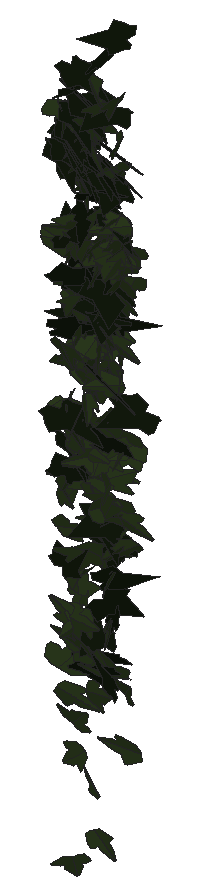
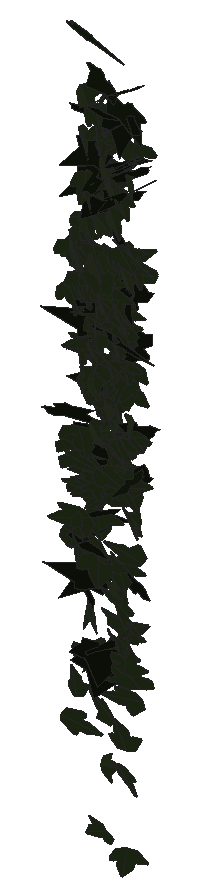
# SketchUp Ruby script. Lengths in millimetres.
U = 1.mm
M = Sketchup.active_model
def pt(a) = Geom::Point3d.new(a.map { |v| v * U })
def face(e, loops, mat)
  f = e.add_face(loops[0].map { |a| pt(a) })
  loops[1..].each { |l| e.add_face(l.map { |a| pt(a) }).erase! }
  f.material = f.back_material = mat if mat
  f
end
# faces: each face lists its corners as indices into pts; further lists are holes
def faces(e, pts, list, mat = nil) = list.each { |f| face(e, (f[0].is_a?(Array) ? f : [f]).map { |l| l.map { |i| pts[i] } }, mat) }
# xy, xz, yz: faces in a plane at the given z, y or x. An outline is a flat list of corners, or four numbers for a rectangle; further outlines are holes
def ring(l) = l.size == 4 ? [[l[0], l[1]], [l[2], l[1]], [l[2], l[3]], [l[0], l[3]]] : l.each_slice(2).to_a
def flat(e, list, mat, &to3) = list.each { |f| face(e, (f[0].is_a?(Array) ? f : [f]).map { |l| ring(l).map { |u, v| to3.(u, v) } }, mat) }
def xy(e, z, list, mat = nil) = flat(e, list, mat) { |x, y| [x, y, z] }
def xz(e, y, list, mat = nil) = flat(e, list, mat) { |x, z| [x, y, z] }
def yz(e, x, list, mat = nil) = flat(e, list, mat) { |y, z| [x, y, z] }
def lines(e, pts, list) = list.each { |a, b| e.add_line(pt(pts[a]), pt(pts[b])) }
# prism: a flat outline (further loops are holes) pulled along v
def prism(e, loops, v, mat = nil)
  f = face(e, loops, mat); d = Geom::Vector3d.new(v.map { |x| x * U })
  f.pushpull(f.normal.samedirection?(d) ? d.length : -d.length)
end
def box(e, o, s, mat = nil) = prism(e, [[o, [o[0] + s[0], o[1], o[2]], [o[0] + s[0], o[1] + s[1], o[2]], [o[0], o[1] + s[1], o[2]]]], [0, 0, s[2]], mat)
def at(x, y, z, deg = 0) = Geom::Transformation.translation(pt([x, y, z])) * Geom::Transformation.rotation(ORIGIN, Z_AXIS, deg.degrees)
def axes(o, x, y, z) = Geom::Transformation.new([*x, 0, *y, 0, *z, 0, *pt(o).to_a, 1])
def part(name) = M.definitions.add(name)
# library, detail: a bought-in or finely detailed component or shape, given as its bounding box
def library(name, o, s) = part(name).tap { |d| box(d.entities, o, s) }
def detail(e, o, s) = box(e.add_group.entities, o, s)
def put(e, d, t, mat = nil) = e.add_instance(d, t).tap { |i| i.material = mat if mat }
def group(e, t, mat = nil) = e.add_group.tap { |g| g.transformation = t; g.material = mat if mat }.entities
root = M.entities
M.materials.add("efeu1").color = [18, 25, 13]
M.materials.add("efeu2").color = [43, 57, 29]
c1 = part("ivyleaf_10")
p = [[0,12.8,-0.8],[-1.5,51.3,-10.9],[-4.9,51,-11.6],[-13.6,26.5,-7.3],[-13.2,15.9,-4.6],[-21.1,19.3,-7.2],
  [-29.5,16.3,-8.3],[-29.2,8.3,-6.2],[-19.7,-9.8,0.5],[-7.6,-13,4],[1,-12.2,5.8],[-0.4,51.1,-11.1],
  [-1.5,51.1,-10.9],[1,-12.4,5.9],[16.9,-12.4,3.5],[35.1,9.1,-5.1],[35,12.9,-6.1],[20.5,16.4,-4.9],
  [15.8,15,-3.8],[15.3,27.6,-7.1],[12.8,31.3,-7.8]]
faces(c1.entities,p,[[0,1,2,3,4,5,6,7,8,9,10],[11,12,0,13,14,15,16,17,18,19,20]],"efeu2")
c2 = part("ivyleaf_9")
p = [[39.1,54.8,31.7],[34.5,51.8,30.2],[-5.3,25.2,17.3],[-17.9,28.3,20.9],[-21.6,21.7,17],[-20.2,4.3,5.3],
  [-22.9,-0.3,2.5],[-17.1,-4,-0.6],[-2,-2.1,-1.2],[-0.7,-15.4,-10.1],[16.6,-22.3,-16.7],[21.1,-15.1,-12.5],
  [32.7,-10.7,-11],[46.1,-1.8,-6.6],[30.8,11.2,3.8]]
faces(c2.entities,p,[[0,1,2,3,4,5,6,7,8,9,10,11,12,13,14]],"efeu1")
put(root,c1,axes([1785.9,1014.5,372.7],[-1.32384,0.17322,0.04012],[0.07345,-0.01106,0.71683],[0.33033,0.69665,0.00141]))
put(root,c1,axes([1792.6,991.7,802.2],[0.13163,0.05618,0.68686],[-0.6877,0.59077,-0.01193],[-1.11685,-0.35715,0.0883]))
put(root,c1,axes([1798.9,996.5,1108.2],[-0.34708,-0.08826,-0.71353],[-0.9192,-0.53026,0.18903],[-1.01363,0.51109,0.0729]))
put(root,c1,axes([1766.4,999.8,777.5],[0.40792,0.09598,-0.63414],[0.94282,0.39989,0.22796],[0.77528,-0.53681,0.05643]))
put(root,c1,axes([1765.5,1006.5,634.8],[0.04265,-0.05749,0.67477],[1.05064,-0.38952,-0.05152],[0.74658,0.55145,0.03395]))
put(root,c1,axes([1789.2,1005,645.7],[0.67204,-0.57726,-0.18258],[-0.18617,0.15419,-0.67669],[1.13715,0.3664,-0.00288]))
put(root,c2,axes([1770.8,1022.5,712.7],[0.27479,-0.73635,0.28054],[0.09446,-0.27615,-0.75037],[1.49672,0.15262,-0.00415]))
put(root,c1,axes([1793.6,1013.7,785.9],[-1.30418,0.02283,0.08212],[-0.15638,-0.00003,-0.68563],[-0.04314,-0.69016,0.00275]))
put(root,c1,axes([1785,1010.7,888.7],[-0.42841,-0.5278,-0.44098],[0.3637,0.39773,-0.57358],[1.25743,-0.29486,0.01566]))
put(root,c2,axes([1776.7,998.5,1241],[-0.01774,-0.77797,0.06994],[0.01085,-0.07001,-0.77799],[1.48656,-0.00877,0.00651]))
put(root,c1,axes([1797.1,1011.5,180.1],[0.83616,-0.46341,-0.33146],[-0.44507,0.23501,-0.63854],[0.98881,0.49766,-0.00712]))
put(root,c2,axes([1802.7,981.4,1102.2],[-1.18914,0.41863,-0.27449],[-0.43994,0.14811,0.75207],[0.84507,0.66618,0.00529]))
put(root,c1,axes([1780.7,998.9,1318.3],[1.35664,0.32212,0.08483],[0.14003,0.04316,-0.78218],[-0.61831,0.71655,0.00898]))
put(root,c1,axes([1790,986.2,904.3],[-1.18737,0.31113,-0.01822],[0.0326,-0.00648,-0.69715],[-0.59225,-0.62411,-0.00184]))
put(root,c1,axes([1793.8,984.5,1095.2],[1.04731,-0.35981,-0.33528],[-0.24813,0.37841,-0.62008],[0.90252,0.52157,0.21859]))
put(root,c1,axes([1792.4,977.6,1313.2],[0.43123,-0.50207,-0.54988],[0.02541,0.57743,-0.52171],[1.41691,0.14245,0.17671]))
put(root,c1,axes([1786.2,1006.2,872.4],[-1.17178,-0.20349,-0.25368],[0.44507,0.10044,-0.64812],[0.43013,-0.65829,-0.02047]))
put(root,c1,axes([1792.3,1007.1,790.6],[1.03405,0.41778,-0.23532],[-0.34769,-0.14845,-0.68535],[-0.84375,0.57318,-0.00598]))
put(root,c2,axes([1778.7,996.7,509.7],[-0.39165,0.4459,0.58644],[0.47429,-0.53086,0.49109],[1.31945,0.32318,-0.00246]))
put(root,c1,axes([1797.7,1009.3,1013.3],[-0.77709,-0.56995,0.02167],[-0.02455,-0.01742,-0.70111],[1.08523,-0.40851,-0.00034]))
put(root,c1,axes([1799,991.3,690.3],[-0.51704,-0.78398,0.10246],[-0.04978,-0.09937,-0.82968],[1.50393,-0.27282,0.00777]))
put(root,c1,axes([1808,995,425],[0.94409,0.16839,0.49544],[-0.89625,-0.15398,0.52384],[0.43419,-0.68397,0.00404]))
put(root,c1,axes([1798.8,1007.2,982.2],[-0.40369,-0.64392,0.20108],[-0.07988,-0.19778,-0.67763],[1.28139,-0.21519,0.02111]))
put(root,c1,axes([1764.1,988,1088],[0.27944,-0.1247,-0.76849],[1.48171,0.02002,0.14549],[-0.00662,-0.78214,0.12625]))
put(root,c1,axes([1773.3,1005.3,571.5],[-0.47828,-0.10464,0.59052],[1.05094,0.20942,0.2721],[-0.44529,0.60664,0.00793]))
put(root,c1,axes([1800.2,1006.5,1120.9],[-0.74213,-0.58021,0.28819],[-0.04439,-0.32357,-0.68301],[1.23217,-0.36112,0.14897]))
put(root,c1,axes([1797,995.8,1262.7],[0.34205,-0.72252,-0.20188],[-0.00346,0.20717,-0.74308],[1.42776,0.1736,0.04656]))
put(root,c1,axes([1799.2,1018.6,782.8],[1.16596,-0.1376,-0.24836],[-0.35791,0.24588,-0.6001],[0.40486,0.61363,0.18476]))
put(root,c1,axes([1797.8,1000.2,1081],[0.28062,-0.72736,0.01988],[0.00687,-0.01956,-0.74215],[1.38481,0.14749,-0.00035]))
put(root,c1,axes([1778.4,999,338.6],[1.38228,0.09781,-0.40417],[0.74656,0.10884,0.73124],[0.26269,-0.82402,0.04861]))
put(root,c1,axes([1787.5,1012.9,231.9],[-1.10305,0.12039,0.3449],[0.64422,-0.06626,0.59194],[0.26146,0.67118,-0.00343]))
put(root,c1,axes([1810.8,1029.3,917.3],[-0.60426,-0.2365,0.57467],[-0.43801,-0.5547,-0.35543],[1.09862,-0.35123,0.17438]))
put(root,c2,axes([1812.9,998.1,1051.4],[0.49239,0.00628,-0.71406],[-1.35077,0.08595,-0.2564],[0.14975,0.7546,0.03515]))
put(root,c1,axes([1799.9,1013.8,924.6],[1.30825,-0.01611,-0.14246],[-0.26758,0.06088,-0.68527],[0.05343,0.69936,0.05637]))
put(root,c1,axes([1803.3,1016.3,1022.3],[0.56734,-0.63795,-0.19127],[-0.15486,0.1731,-0.70416],[1.25805,0.30901,-0.00042]))
put(root,c1,axes([1800.9,1020.6,860.8],[0.69108,-0.56114,-0.19193],[-0.05014,0.20956,-0.66254],[1.12758,0.35323,0.08817]))
put(root,c1,axes([1792.5,1008,779.3],[0.83922,-0.38423,0.29154],[0.40064,-0.2021,-0.58473],[0.8259,0.48846,-0.0126]))
put(root,c1,axes([1801.1,1004.8,413.4],[-0.20224,-0.15516,0.71497],[0.18983,-0.7188,-0.14117],[1.37941,0.07617,0.12425]))
put(root,c1,axes([1808.6,1023.7,1026.1],[-0.75326,-0.54105,0.26057],[-0.12857,-0.26997,-0.6632],[1.13567,-0.38943,0.09775]))
put(root,c1,axes([1803.4,1006.4,477.5],[1.25925,-0.25225,0.22653],[-0.39329,0.09376,0.70798],[-0.51155,-0.69304,0.01333]))
put(root,c2,axes([1816.2,980.4,1370.1],[-0.07001,0.77537,0.07741],[-0.19552,0.072,-0.76994],[-1.47007,-0.0465,0.09871]))
put(root,c2,axes([1807.7,994.1,1355.5],[1.00357,0.07387,-0.59041],[-1.13062,0.10985,-0.51683],[0.06387,0.78394,0.12805]))
put(root,c1,axes([1801.9,1014.9,737.3],[-0.78919,0.56043,0.30811],[0.28524,-0.27183,0.69614],[1.18328,0.4393,0.03769]))
put(root,c1,axes([1799.7,1005.8,783],[0.64562,-0.65328,0.32352],[0.24317,-0.29803,-0.73578],[1.36595,0.36183,-0.02193]))
put(root,c1,axes([1820.8,980.6,743.9],[-0.41521,0.25712,-0.62747],[-0.7233,0.49953,0.33683],[1.06883,0.43792,-0.01581]))
put(root,c2,axes([1793,1001.6,1278.8],[-0.0433,-0.7828,0.01386],[-0.02321,-0.01351,-0.78304],[1.48988,-0.02296,-0.01179]))
put(root,c1,axes([1816.8,1008.6,670.1],[0.18627,0.35208,0.67435],[-0.52245,-0.61775,0.36237],[1.35026,-0.28759,0.04719]))
put(root,c1,axes([1794.6,1004.7,1021.5],[-0.00977,-0.50341,0.5644],[0.26754,0.55394,0.49536],[-1.41427,0.10827,0.08981]))
put(root,c2,axes([1792.9,989,1262.8],[0.11086,-0.68428,-0.36084],[-0.0587,0.35952,-0.68675],[1.47113,0.06591,-0.00021]))
put(root,c1,axes([1808.9,1018.9,1191.8],[0.07276,-0.7428,-0.0518],[-0.02022,0.05132,-0.74374],[1.41699,0.03887,-0.00796]))
put(root,c1,axes([1807.4,1007.5,913.9],[-0.2,-0.60885,-0.37772],[0.09736,0.37441,-0.61775],[1.36016,-0.11633,-0.01132]))
put(root,c1,axes([1814.7,999.1,541.8],[-1.22595,-0.35748,0.14599],[-0.2251,-0.08764,-0.73645],[0.69958,-0.65465,0.01888]))
put(root,c1,axes([1804.1,1009.5,910.5],[0.17045,0.58033,-0.46299],[-0.15794,-0.4556,-0.58712],[-1.40407,0.1217,0.00984]))
put(root,c1,axes([1829.6,986.3,376.8],[-0.21957,0.08073,-0.70751],[-1.06936,0.43,0.14069],[0.8326,0.57357,-0.00589]))
put(root,c2,axes([1792.4,1003.3,1228.2],[0.19118,-0.61787,-0.45979],[0.04473,0.46593,-0.62098],[1.46512,0.0664,0.07895]))
put(root,c2,axes([1794.5,1000.2,1285.8],[0.07838,-0.78587,-0.00932],[-0.00057,0.00932,-0.78695],[1.49578,0.04118,0.00019]))
put(root,c2,axes([1802.6,1001.4,1282.4],[-0.5311,-0.73042,0.00033],[-0.00889,0.00144,-0.78189],[1.3901,-0.27905,-0.00487]))
put(root,c2,axes([1789.6,981.2,795.1],[0.09595,-0.48785,-0.65914],[0.28899,0.65451,-0.47282],[1.5337,-0.09281,0.13033]))
put(root,c1,axes([1805.8,1006.6,470],[0.96861,-0.53914,0.06018],[0.09057,-0.03784,-0.74136],[1.02849,0.51109,0.0086]))
put(root,c2,axes([1836.7,1010.8,960.9],[-1.16513,0.27363,0.39767],[-0.69022,0.16314,-0.67056],[-0.6063,-0.71155,-0.00082]))
put(root,c1,axes([1818.4,1017,1045.6],[-1.27466,-0.13316,0.18494],[-0.32662,-0.08305,-0.68128],[0.28537,-0.68983,0.04633]))
put(root,c1,axes([1809.7,982.4,9.3],[-0.77648,-0.54294,-0.15661],[0.18239,0.12388,-0.67914],[1.05987,-0.41909,0.00214]))
put(root,c2,axes([1797.6,979.5,686.6],[-0.34207,-0.10602,0.805],[1.2958,0.42953,0.20858],[-0.84193,0.70415,-0.00604]))
put(root,c1,axes([1820,1005.4,963.9],[-1.26971,-0.13294,0.192],[-0.35032,-0.05831,-0.67995],[0.27354,-0.69177,0.02042]))
put(root,c1,axes([1810.9,1010.6,414.5],[0.94085,-0.48104,-0.05138],[-0.06618,0.03795,-0.68976],[0.91834,0.49557,0.00294]))
put(root,c1,axes([1814.4,994.5,1220.5],[1.01857,-0.45649,-0.30923],[-0.23845,0.31899,-0.68774],[1.02192,0.52943,0.14774]))
put(root,c2,axes([1786.1,976.8,940.2],[0.64113,0.10623,0.71943],[1.28956,0.24209,-0.35302],[-0.50265,0.7566,0.01195]))
put(root,c1,axes([1809.9,1003.8,939.3],[0.33519,-0.66475,0.24323],[0.19875,-0.2235,-0.68645],[1.33245,0.20056,0.04121]))
put(root,c1,axes([1805.2,1021.5,822.8],[-0.68534,0.50791,-0.20045],[0.24598,-0.15401,-0.62241],[-1.00968,-0.38227,-0.01558]))
put(root,c1,axes([1823.8,1021.3,716.7],[-0.51332,-0.44167,0.43769],[-0.43012,-0.37484,-0.5175],[1.10249,-0.35188,0.00189]))
put(root,c1,axes([1808.4,1029.7,852.5],[0.21638,-0.54458,0.41217],[0.31279,-0.38375,-0.55236],[1.26163,0.18854,0.06626]))
put(root,c1,axes([1813.3,1017.5,1036.8],[-0.61788,-0.59833,-0.18138],[0.21842,0.14388,-0.68002],[1.1697,-0.34293,0.03117]))
put(root,c1,axes([1816,1018.8,844.4],[0.59184,0.62116,0.04643],[-0.085,-0.02952,0.69414],[1.18243,-0.31303,0.02666]))
put(root,c1,axes([1807.2,1005.4,496.8],[-0.1283,-0.53735,-0.38146],[0.12273,-0.38699,0.53375],[-1.24816,0.01718,0.09169]))
put(root,c2,axes([1793.6,981.2,1025],[0.03381,-0.08125,0.79188],[1.42347,0.27285,0.01122],[-0.51863,0.7436,0.08241]))
put(root,c1,axes([1789.6,1009.7,988.6],[0.80175,-0.0179,0.59278],[1.12853,0.02479,-0.42065],[-0.01874,0.7268,0.02895]))
put(root,c1,axes([1813.8,1025.5,831.8],[0.70803,-0.56833,0.05113],[0.06133,-0.04001,-0.67924],[1.08427,0.37338,0.00503]))
put(root,c1,axes([1792.2,986.5,298.3],[-0.44925,0.00003,-0.6743],[1.23846,-0.18727,-0.2278],[-0.33641,-0.68945,0.06184]))
put(root,c2,axes([1802.2,994.7,1320.5],[0.19585,-0.7898,0.02099],[0.00477,-0.02084,-0.79648],[1.50368,0.10293,-0.00021]))
put(root,c1,axes([1804.2,1021.4,754.2],[0.90796,-0.32733,0.41814],[0.63362,-0.25354,-0.57833],[0.78736,0.58151,-0.01678]))
put(root,c1,axes([1820.4,1018,1110.5],[-0.1513,-0.67236,0.28448],[0.03792,-0.28805,-0.67524],[1.38895,-0.06537,0.04943]))
put(root,c1,axes([1820,992.7,1244.7],[-0.07251,-0.71019,-0.293],[0.08396,0.29085,-0.71073],[1.45974,-0.05201,0.02632]))
put(root,c1,axes([1830.5,999.8,718.8],[0.1528,0.14766,-0.67656],[-0.83484,-0.51618,-0.16471],[-1.01981,0.44468,0.03346]))
put(root,c1,axes([1791.7,995.4,426.8],[0.15242,-0.14421,-0.82456],[1.21966,-0.52234,0.1536],[-1.02494,-0.64302,0.06016]))
put(root,c1,axes([1824.9,1025.7,1035.6],[0.16205,-0.70553,0.10179],[0.03598,-0.10024,-0.71062],[1.35619,0.08696,0.00669]))
put(root,c1,axes([1827.7,999,1093.8],[-0.40716,-0.69356,0.05873],[-0.02987,-0.05662,-0.72581],[1.32438,-0.2145,0.00168]))
put(root,c1,axes([1827.9,1014.5,1035.2],[-1.16691,-0.34505,-0.01618],[0.03502,0.00029,-0.7035],[0.65648,-0.61334,0.00877]))
put(root,c1,axes([1826.5,1013,892.9],[0.04915,-0.65439,-0.26144],[0.07265,0.26253,-0.65335],[1.33918,0.00978,0.04504]))
put(root,c1,axes([1798.9,1003.1,727.8],[-0.14766,-0.05338,-0.76196],[1.27924,-0.36856,-0.04262],[-0.69051,-0.67138,0.08398]))
put(root,c2,axes([1807.4,985.9,1406.1],[0.48938,-0.63486,-0.4056],[0.09205,0.44161,-0.66055],[1.43085,0.18873,0.18122]))
put(root,c2,axes([1827.3,1027.7,401.9],[-0.59266,-0.63437,0.37839],[-0.32314,-0.33817,-0.70667],[1.36815,-0.35467,-0.003]))
put(root,c2,axes([1849,996.7,1017.4],[-0.37812,0.44998,0.63914],[-0.51517,0.57905,-0.49181],[-1.39558,-0.33567,0.00838]))
put(root,c1,axes([1834,999.3,679.4],[-0.29699,0.4272,0.60679],[-0.53472,0.53989,-0.45236],[-1.30721,-0.31791,0.04718]))
put(root,c1,axes([1826.5,1005.3,1242.6],[0.27828,-0.70765,0.31109],[0.21624,-0.29349,-0.72102],[1.45521,0.17894,0.04765]))
put(root,c2,axes([1824.9,994.6,1150.3],[-0.95984,0.15283,-0.57285],[1.04871,-0.15676,-0.52693],[-0.41647,-0.74695,-0.00662]))
put(root,c1,axes([1831.9,1009.4,1274],[0.07091,-0.76654,-0.001],[0.00001,0.001,-0.76744],[1.45888,0.03726,0.00005]))
put(root,c1,axes([1801.5,1015.5,912.4],[-0.02851,-0.10325,0.72326],[1.38708,0.04832,0.02199],[-0.09693,0.7218,0.10199]))
put(root,c1,axes([1836.8,1021.2,1070.8],[-1.10884,-0.45077,0.07123],[-0.12646,-0.0305,-0.73646],[0.8593,-0.58617,-0.01646]))
put(root,c1,axes([1840.8,1017.8,847],[-1.00728,0.30414,0.26947],[-0.55613,0.02262,-0.59944],[-0.5374,-0.59348,0.11525]))
put(root,c1,axes([1833.2,1004.6,852.5],[-1.51867,0.05913,-0.01521],[0.02799,-0.00737,-0.80012],[-0.11277,-0.79807,0.00626]))
put(root,c1,axes([1836.3,976,1198.9],[0.63003,-0.35753,-0.58055],[-0.22082,0.60641,-0.43961],[1.2787,0.28088,0.21013]))
put(root,c1,axes([1810.7,1029.3,283.7],[0.39325,-0.22156,-0.6991],[0.82069,-0.55079,0.30201],[-1.12898,-0.47756,-0.02398]))
put(root,c1,axes([1823.8,997.8,906.2],[0.67494,0.40319,-0.45112],[0.44121,0.39245,0.53299],[1.06363,-0.41864,0.06517]))
put(root,c2,axes([1816.7,998.2,1341.9],[0.30127,-0.75586,-0.16787],[-0.00636,0.17067,-0.77164],[1.47359,0.15527,0.03099]))
put(root,c1,axes([1836.6,1020,552.4],[-1.19105,-0.54341,-0.04469],[0.06541,0.02858,-0.82881],[1.03564,-0.62676,0.00095]))
put(root,c1,axes([1818.9,1026.2,922.2],[1.04545,-0.26189,0.33521],[0.60895,-0.1064,-0.60745],[0.53349,0.63465,0.03649]))
put(root,c2,axes([1824,996.7,1247.1],[-0.21591,-0.7558,0.01866],[-0.00432,-0.01852,-0.76427],[1.43887,-0.11347,0.00051]))
put(root,c1,axes([1856.2,1006.1,1065.5],[-0.82089,0.07761,0.56223],[-1.01998,-0.28817,-0.37136],[0.3556,-0.64739,0.23271]))
put(root,c1,axes([1830.7,990,822.9],[-0.03201,0.64786,-0.29071],[-0.02227,-0.291,-0.64784],[-1.35126,-0.01055,0.01756]))
put(root,c1,axes([1842.5,1011.4,866.1],[-0.06205,-0.63607,0.3329],[0.00516,-0.33335,-0.63667],[1.36634,-0.02763,0.01753]))
put(root,c1,axes([1842.2,989.2,1315.2],[-1.29402,-0.37141,-0.06905],[0.11537,0.03305,-0.77475],[0.70966,-0.68262,0.00005]))
put(root,c2,axes([1845.1,994.8,1415.8],[-0.65979,0.56148,-0.44715],[-0.42785,0.38665,0.65981],[1.29734,0.41307,-0.00981]))
put(root,c1,axes([1843.8,998.9,1101],[0.23371,-0.72769,0.01937],[0.00309,-0.01937,-0.73798],[1.38543,0.1228,-0.00162]))
put(root,c2,axes([1838.2,994.1,352.7],[1.22001,0.44977,-0.1962],[-0.30171,-0.11566,-0.78307],[-0.88383,0.66033,-0.00352]))
put(root,c1,axes([1819.3,1008.5,1070.7],[-0.39028,-0.00416,0.72934],[1.27203,-0.30435,0.18619],[0.55566,0.6938,0.08605]))
put(root,c2,axes([1843.3,999,375.1],[0.95766,0.52901,-0.2124],[-0.30304,-0.14161,-0.7299],[-1.04175,0.5275,0.01707]))
put(root,c1,axes([1845.9,1019.4,1099],[-0.043,-0.74387,0.01041],[0.005,-0.01049,-0.74421],[1.41586,-0.02255,0.00294]))
put(root,c1,axes([1857.7,975,151.4],[-0.31331,0.31635,-0.57425],[-0.52824,0.50277,0.35654],[1.13044,0.32262,0.00745]))
put(root,c1,axes([1846.5,1019.1,791.3],[0.19069,-0.65783,0.16168],[0.03809,-0.1605,-0.66541],[1.28869,0.10208,-0.00426]))
put(root,c1,axes([1846.3,1020.2,878.4],[0.00518,-0.62912,0.27947],[0.10508,-0.27837,-0.62719],[1.30594,0.0249,0.04936]))
put(root,c1,axes([1848.8,987.5,1055],[0.32437,-0.69045,-0.23697],[-0.04267,0.23827,-0.71038],[1.38864,0.1686,0.03352]))
put(root,c2,axes([1864.4,1012.6,1004.3],[-0.29481,-0.05537,0.76654],[-1.2885,-0.36023,-0.16284],[0.69222,-0.69412,0.02336]))
put(root,c1,axes([1842.8,1005.5,725.4],[1.42983,-0.00861,-0.03698],[-0.07021,0.00752,-0.75129],[0.01707,0.75215,0.00708]))
put(root,c1,axes([1856.4,1012.7,1108.9],[-1.35202,0.08947,0.19301],[-0.37732,-0.03442,-0.71374],[-0.14684,-0.73534,0.05689]))
put(root,c2,axes([1838.5,1002.8,1224.9],[-0.10928,-0.66271,0.37873],[-0.04551,-0.37806,-0.66515],[1.45199,-0.06173,0.00766]))
put(root,c1,axes([1838.6,1032.6,928.7],[-0.32453,0.14806,-0.64034],[0.35934,-0.62262,-0.19424],[-1.19813,-0.22684,0.11519]))
put(root,c1,axes([1856.1,999.1,618.4],[-1.04614,-0.45949,0.07673],[-0.11496,-0.04738,-0.71643],[0.87913,-0.55298,-0.00238]))
put(root,c1,axes([1823.9,1008.3,771.3],[0.63406,-0.06117,0.66451],[1.26961,0.01131,-0.33341],[0.03286,0.74326,0.05976]))
put(root,c1,axes([1829.4,1023.7,575.6],[0.69009,-0.17479,0.55642],[1.05152,-0.10693,-0.39363],[0.35556,0.65548,0.08416]))
put(root,c1,axes([1841.9,1005.4,911.8],[0.39026,-0.45579,0.53559],[0.58666,-0.4432,-0.49518],[1.20306,0.36397,0.06773]))
put(root,c1,axes([1852.3,1001.8,991.2],[0.10509,-0.62858,-0.35205],[0.11183,0.35584,-0.62612],[1.3666,0.01922,0.07831]))
put(root,c1,axes([1832.1,997.4,1268.6],[0.51448,-0.38703,0.60995],[1.04193,-0.31514,-0.44259],[0.89697,0.58805,0.16426]))
put(root,c1,axes([1833.8,1019.8,967.5],[-0.46904,0.21969,-0.6494],[0.82655,-0.48392,-0.32853],[-1.00955,-0.49827,0.03274]))
put(root,c1,axes([1831.8,1003.5,952.7],[-0.77265,0.0357,0.61102],[1.1617,-0.03049,0.40734],[0.08597,0.73296,-0.01282]))
put(root,c2,axes([1865.6,1002.6,614.7],[-0.90892,-0.42822,0.46382],[-0.66807,-0.30324,-0.6414],[0.99855,-0.59266,-0.00694]))
put(root,c1,axes([1838.8,1015,684.1],[-0.8536,-0.13524,-0.49031],[0.89142,0.14502,-0.46845],[0.37736,-0.64848,-0.00251]))
put(root,c1,axes([1844.2,1020.8,885.2],[-0.82403,0.37171,-0.35765],[0.45967,-0.2665,-0.56937],[-0.86747,-0.49432,0.03803]))
put(root,c1,axes([1847.8,998.8,989.1],[-1.14122,-0.23915,-0.27782],[0.5303,0.04875,-0.64336],[0.45333,-0.65906,0.05322]))
put(root,c1,axes([1854.2,993.8,1156.2],[0.06438,-0.63617,0.40051],[0.17458,-0.39443,-0.63425],[1.42003,0.07733,0.05982]))
put(root,c2,axes([1863.2,995.6,766.1],[0.94249,0.23706,-0.52645],[-0.91281,-0.21721,-0.54897],[-0.61172,0.68935,0.00807]))
put(root,c1,axes([1853,979.6,1389.3],[-0.42787,0.76053,0.0821],[-0.05045,0.07777,-0.79305],[-1.45497,-0.22635,0.00336]))
put(root,c1,axes([1866.3,1000.1,351.7],[-1.39313,-0.18456,-0.21761],[-0.39268,-0.07149,0.75468],[-0.37511,0.7603,0.01813]))
put(root,c2,axes([1843,1019.7,597.4],[0.09079,-0.81547,0.17255],[0.03635,-0.17172,-0.81681],[1.58594,0.05062,0.00884]))
put(root,c1,axes([1863.6,993.4,1351.8],[-0.41024,-0.7521,0.12961],[-0.05125,-0.1271,-0.78232],[1.45158,-0.21704,0.00901]))
put(root,c1,axes([1860.4,992,1324.1],[0.61092,-0.63192,-0.37242],[-0.0275,0.40099,-0.69286],[1.39573,0.2845,0.14936]))
put(root,c1,axes([1834.7,1015.2,690.9],[-0.35156,-0.05142,-0.72029],[1.33418,0.16566,-0.19161],[0.32983,-0.72491,0.0073]))
put(root,c1,axes([1839,1004.4,50.4],[0.7558,-0.09392,0.50944],[0.9527,-0.09561,-0.40784],[0.25371,0.63882,0.01386]))
put(root,c1,axes([1858.1,978.3,643.8],[0.0614,0.0851,0.77042],[-0.18284,0.76558,-0.08055],[-1.46381,-0.09206,0.04237]))
put(root,c2,axes([1846.7,1005.5,1240.2],[0.02866,-0.74074,0.19515],[0.08164,-0.19407,-0.73993],[1.45559,0.02547,0.03766]))
put(root,c2,axes([1851.7,977,1199.7],[1.07706,0.49019,0.12833],[0.19419,0.0782,-0.74866],[-0.94462,0.57499,-0.00758]))
put(root,c1,axes([1877,1000.7,861.2],[-0.23613,-0.02979,0.65734],[-0.58963,-0.58749,-0.0851],[1.10484,-0.3199,0.09508]))
put(root,c2,axes([1861.2,999.8,992.2],[-0.81312,-0.61226,-0.13834],[0.14551,0.11534,-0.74658],[1.18574,-0.43401,-0.00325]))
put(root,c1,axes([1866,1002.6,1182.5],[0.43395,-0.734,-0.06651],[0.00648,0.07067,-0.76822],[1.40266,0.22676,0.02413]))
put(root,c1,axes([1844.3,988.7,677.1],[-0.62571,-0.02586,-0.57333],[1.05384,-0.18805,-0.30904],[-0.28723,-0.63359,0.11512]))
put(root,c2,axes([1862.6,1023.4,577.3],[-1.20033,-0.076,-0.43592],[0.81916,0.07082,-0.63507],[0.19549,-0.7634,-0.01552]))
put(root,c1,axes([1869.1,1021.3,1057.7],[-0.93654,-0.52091,-0.02258],[0.02848,0.01693,-0.71659],[0.99192,-0.49232,-0.00074]))
put(root,c2,axes([1877.3,997.8,1353.5],[-1.44072,-0.21652,-0.02581],[0.08582,-0.06421,-0.78386],[0.40603,-0.75471,0.07409]))
put(root,c1,axes([1867.8,1005.8,447.9],[0.04784,-0.42239,-0.48291],[0.07294,0.4834,-0.42083],[1.21886,-0.01235,0.04414]))
put(root,c2,axes([1841.2,998.4,871.5],[0.90119,-0.63218,0.24455],[0.31578,-0.18113,-0.78952],[1.25081,0.50121,0.02313]))
put(root,c1,axes([1872,1006.3,1229.2],[-0.11396,-0.65964,0.38728],[-0.06074,-0.38597,-0.66234],[1.45453,-0.0678,0.00268]))
put(root,c1,axes([1874.7,1027,606.3],[-0.03925,-0.0121,-0.69439],[-0.59259,-0.62081,0.02006],[-1.18149,0.31177,0.013]))
put(root,c1,axes([1868.8,1012.6,1236.2],[-0.58541,-0.67798,-0.25733],[0.20714,0.2332,-0.74449],[1.36453,-0.32627,0.00262]))
put(root,c1,axes([1865.9,1011.7,942.3],[0.50883,0.70399,-0.16882],[-0.15211,-0.15016,-0.75276],[-1.3694,0.27826,0.02089]))
put(root,c2,axes([1864.3,999.9,1025.6],[-0.84007,-0.55364,-0.28117],[0.32348,0.22407,-0.70803],[1.13665,-0.47295,-0.00631]))
put(root,c1,axes([1867.2,1004,520.3],[0.45442,-0.56585,0.25066],[0.16799,-0.23479,-0.61409],[1.16582,0.25439,-0.00921]))
put(root,c1,axes([1868.7,983.3,958.8],[-0.83072,0.55166,0.04397],[-0.0532,0.03394,-0.70345],[-1.0519,-0.43738,0.00086]))
put(root,c2,axes([1849.7,995.8,1241.3],[0.38212,-0.66191,0.37994],[0.23166,-0.36006,-0.69161],[1.43393,0.23456,0.01048]))
put(root,c2,axes([1853.3,1009.3,1241.5],[1.22971,-0.3981,-0.21204],[-0.27723,0.16642,-0.75631],[0.81243,0.65935,0.06287]))
put(root,c1,axes([1880.4,1015.6,769.8],[-1.30472,-0.14741,0.18921],[-0.35249,-0.0387,-0.70121],[0.29006,-0.71012,-0.00106]))
put(root,c1,axes([1876.4,980.2,693.1],[0.52782,-0.58945,-0.42413],[-0.21272,0.41395,-0.64839],[1.3656,0.29231,0.06293]))
put(root,c1,axes([1872.4,1000.7,1131.8],[0.4694,-0.66818,-0.19615],[0.00077,0.20823,-0.70881],[1.32534,0.23653,0.06988]))
put(root,c1,axes([1887.7,1006,1045.3],[-1.05567,0.25186,0.41986],[-0.77429,0.11589,-0.60699],[-0.51843,-0.68594,0.05161]))
put(root,c1,axes([1884.3,1027.7,728.7],[0.68236,0.26653,-0.51125],[-0.87274,-0.23309,-0.44311],[-0.66511,0.5793,0.05692]))
put(root,c1,axes([1866.2,1003.2,434.2],[0.54626,-0.56409,0.40028],[0.40289,-0.34093,-0.63226],[1.25323,0.35548,0.02879]))
put(root,c2,axes([1882.8,987.9,336.4],[-0.06563,-0.70959,0.40892],[0.11206,0.40607,0.70961],[-1.55464,0.05923,0.03389]))
put(root,c2,axes([1853,993.9,1283.3],[1.4014,-0.23569,-0.03729],[-0.01614,0.09504,-0.76813],[0.45386,0.73113,0.08783]))
put(root,c1,axes([1883.6,988.7,664.4],[-1.32385,-0.32197,0.17383],[-0.29977,-0.07355,-0.76649],[0.62855,-0.7132,0.00057]))
put(root,c1,axes([1878.3,1010.8,1040],[0.12887,-0.74584,-0.01934],[-0.009,0.01899,-0.7489],[1.41992,0.06781,-0.00299]))
put(root,c1,axes([1875.8,1018.8,1064.8],[0.67494,-0.63594,0.00442],[0.03407,0.00492,-0.72791],[1.20986,0.35463,0.01803]))
put(root,c1,axes([1867.4,1025,862.3],[0.52855,-0.47561,0.42894],[0.48401,-0.3472,-0.54963],[1.11871,0.37492,0.03514]))
put(root,c1,axes([1877.9,1013.9,914.6],[0.56703,-0.53992,-0.35051],[-0.03855,0.37818,-0.59975],[1.22452,0.26192,0.14343]))
put(root,c1,axes([1880.2,998.3,1153.7],[-0.09032,-0.73603,-0.09381],[0.007,0.09377,-0.73755],[1.41213,-0.04754,-0.00235]))
put(root,c2,axes([1887.6,983.3,451.1],[0.00571,0.00331,0.81473],[0.01043,0.81472,-0.00333],[-1.55058,0.00549,0.00298]))
put(root,c2,axes([1875.3,998.8,1219.7],[-0.64134,-0.68499,0.15608],[-0.01495,-0.16943,-0.7605],[1.33701,-0.33048,0.06637]))
put(root,c1,axes([1892.2,997.5,1148.6],[-0.39592,-0.01437,0.71782],[-0.49378,-0.69533,-0.08911],[1.27408,-0.27395,0.18853]))
put(root,c1,axes([1861.1,1010.1,932.2],[-0.80687,0.08711,-0.54663],[0.99462,-0.16393,-0.43144],[-0.34719,-0.67206,0.03439]))
put(root,c2,axes([1905.2,987.9,1487.7],[-1.1023,0.55506,0.11718],[-0.35818,-0.03002,-0.78801],[-1.01853,-0.59015,0.1503]))
put(root,c1,axes([1884.2,994.6,1086.3],[-0.47831,-0.6333,0.30957],[0.03087,-0.33376,-0.66963],[1.34123,-0.21816,0.12581]))
put(root,c1,axes([1881.8,1022.4,1101.6],[0.61662,-0.64747,-0.0028],[-0.00368,0.00217,-0.72401],[1.23227,0.324,-0.00076]))
put(root,c2,axes([1865.9,1004.5,1157.8],[0.29396,-0.74118,-0.1195],[0.00606,0.12265,-0.75659],[1.42881,0.15197,0.02779]))
put(root,c1,axes([1884.7,1007.4,572.3],[-0.23553,-0.68789,-0.34855],[0.05926,0.34827,-0.69838],[1.46647,-0.12455,-0.02776]))
put(root,c1,axes([1885.7,999.3,740.1],[0.41894,-0.63361,-0.1607],[-0.12279,0.14768,-0.67065],[1.23799,0.22906,-0.01214]))
put(root,c2,axes([1858.3,1002.7,506.8],[0.32581,0.07478,0.74828],[1.36896,0.20761,-0.18531],[-0.41755,0.739,-0.02366]))
put(root,c1,axes([1884.6,1004.4,1014.3],[-1.09948,0.40607,0.05433],[-0.0912,0.02631,-0.70612],[-0.77438,-0.57966,0.00601]))
put(root,c1,axes([1875,1026.4,306.4],[-0.90683,0.28019,0.39589],[0.6186,-0.22744,0.55217],[0.68513,0.57622,0.02544]))
put(root,c1,axes([1903.6,1009.7,1096.8],[0.1463,0.06986,-0.77003],[-0.95037,0.59529,0.00416],[1.12349,0.49446,0.10379]))
put(root,c2,axes([1855.6,995.3,965.9],[0.51922,0.02659,0.75816],[1.43568,0.0759,-0.27411],[-0.15304,0.80217,0.00081]))
put(root,c1,axes([1887.2,1020.7,1112.1],[0.23487,-0.7267,-0.07436],[0.00496,0.07586,-0.73695],[1.39027,0.1225,0.01519]))
put(root,c1,axes([1866.8,993.3,1098.8],[-0.63458,-0.28876,-0.59565],[1.10743,0.19011,-0.41788],[0.60062,-0.65561,0.14117]))
put(root,c1,axes([1895.4,1021.7,751.3],[0.67649,0.30668,-0.53779],[-0.76251,-0.35881,-0.46942],[-0.89826,0.53555,-0.00654]))
put(root,c1,axes([1890.7,1027.8,1036.8],[-0.6668,-0.59755,0.21177],[0.00291,-0.24276,-0.68244],[1.20656,-0.32965,0.11868]))
put(root,c1,axes([1899.6,1010.4,579.3],[-0.3855,-0.43999,0.57486],[-0.48116,-0.51636,-0.48429],[1.291,-0.32383,-0.00884]))
put(root,c1,axes([1910.9,998.9,228.8],[0.19473,0.00181,-0.71091],[-1.25792,0.26474,-0.09446],[0.49825,0.66766,0.03938]))
put(root,c2,axes([1879,974.6,495.4],[0.01907,-0.07622,-0.85856],[-0.28109,0.84576,-0.07681],[1.61617,0.148,-0.00323]))
put(root,c1,axes([1891.6,987.8,1374.8],[-0.06946,-0.80712,0.01247],[-0.00278,-0.01242,-0.80794],[1.53629,-0.03651,-0.0009]))
put(root,c1,axes([1890.5,992.9,1300.4],[0.35057,-0.76303,-0.14466],[-0.00981,0.14747,-0.78441],[1.47804,0.18196,0.02911]))
put(root,c1,axes([1892.9,996.3,1122.9],[-0.29651,-0.72339,-0.16286],[0.03126,0.16301,-0.73976],[1.41086,-0.15564,-0.01784]))
put(root,c2,axes([1908.1,1031,810.8],[-1.33781,-0.27658,0.27252],[-0.48358,-0.09853,-0.75538],[0.55879,-0.74744,-0.00127]))
put(root,c1,axes([1868.5,999.5,694.3],[0.95608,-0.11842,-0.47931],[0.91002,-0.05369,0.5144],[-0.23412,-0.69226,0.0421]))
put(root,c1,axes([1888.7,1007,1104.5],[-0.68512,0.64639,0.04082],[-0.04199,0.03443,-0.73987],[-1.23195,-0.36065,0.00252]))
put(root,c1,axes([1897.9,1009.5,1102.6],[-1.04979,-0.45539,0.08035],[-0.11292,-0.05433,-0.71527],[0.8728,-0.55476,0.0041]))
put(root,c1,axes([1898.5,1004.7,1108.1],[-0.12874,0.20523,-0.7114],[-0.5052,-0.6736,-0.16908],[-1.31547,0.2386,0.13456]))
put(root,c1,axes([1872.4,1019.8,620],[-0.8393,0.08158,-0.5989],[1.12379,-0.10023,-0.44844],[-0.24575,-0.73696,-0.00531]))
